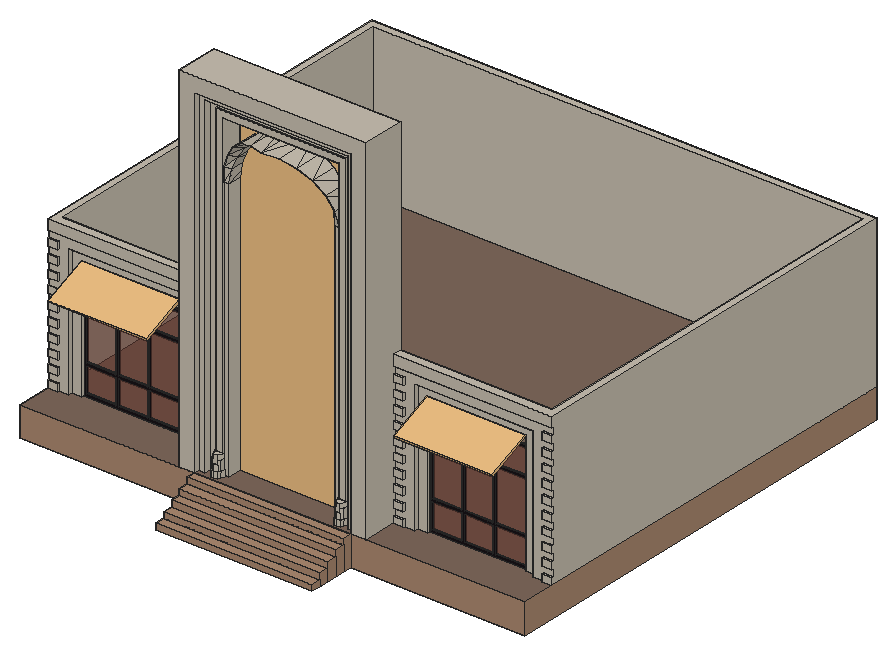
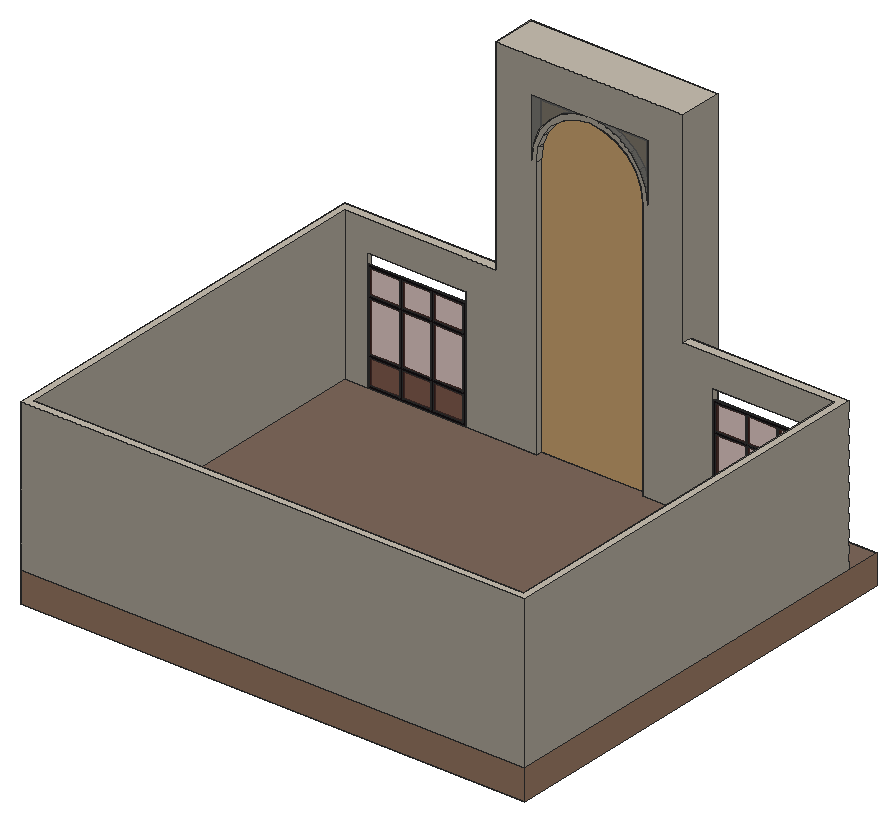
# SketchUp Ruby script. Lengths in inches.
U = 1.inch
M = Sketchup.active_model
def pt(a) = Geom::Point3d.new(a.map { |v| v * U })
def face(e, loops, mat)
  f = e.add_face(loops[0].map { |a| pt(a) })
  loops[1..].each { |l| e.add_face(l.map { |a| pt(a) }).erase! }
  f.material = f.back_material = mat if mat
  f
end
# faces: each face lists its corners as indices into pts; further lists are holes
def faces(e, pts, list, mat = nil) = list.each { |f| face(e, (f[0].is_a?(Array) ? f : [f]).map { |l| l.map { |i| pts[i] } }, mat) }
# xy, xz, yz: faces in a plane at the given z, y or x. An outline is a flat list of corners, or four numbers for a rectangle; further outlines are holes
def ring(l) = l.size == 4 ? [[l[0], l[1]], [l[2], l[1]], [l[2], l[3]], [l[0], l[3]]] : l.each_slice(2).to_a
def flat(e, list, mat, &to3) = list.each { |f| face(e, (f[0].is_a?(Array) ? f : [f]).map { |l| ring(l).map { |u, v| to3.(u, v) } }, mat) }
def xy(e, z, list, mat = nil) = flat(e, list, mat) { |x, y| [x, y, z] }
def xz(e, y, list, mat = nil) = flat(e, list, mat) { |x, z| [x, y, z] }
def yz(e, x, list, mat = nil) = flat(e, list, mat) { |y, z| [x, y, z] }
def lines(e, pts, list) = list.each { |a, b| e.add_line(pt(pts[a]), pt(pts[b])) }
# prism: a flat outline (further loops are holes) pulled along v
def prism(e, loops, v, mat = nil)
  f = face(e, loops, mat); d = Geom::Vector3d.new(v.map { |x| x * U })
  f.pushpull(f.normal.samedirection?(d) ? d.length : -d.length)
end
def box(e, o, s, mat = nil) = prism(e, [[o, [o[0] + s[0], o[1], o[2]], [o[0] + s[0], o[1] + s[1], o[2]], [o[0], o[1] + s[1], o[2]]]], [0, 0, s[2]], mat)
def at(x, y, z, deg = 0) = Geom::Transformation.translation(pt([x, y, z])) * Geom::Transformation.rotation(ORIGIN, Z_AXIS, deg.degrees)
def axes(o, x, y, z) = Geom::Transformation.new([*x, 0, *y, 0, *z, 0, *pt(o).to_a, 1])
def part(name) = M.definitions.add(name)
# library, detail: a bought-in or finely detailed component or shape, given as its bounding box
def library(name, o, s) = part(name).tap { |d| box(d.entities, o, s) }
def detail(e, o, s) = box(e.add_group.entities, o, s)
def put(e, d, t, mat = nil) = e.add_instance(d, t).tap { |i| i.material = mat if mat }
def group(e, t, mat = nil) = e.add_group.tap { |g| g.transformation = t; g.material = mat if mat }.entities
root = M.entities
M.materials.add("[0034_Wheat]").color = [198, 190, 175]
M.materials.add("[Color M06]").color = [86, 86, 86]
M.materials.add("[Color M07]").color = [25, 20, 24]
M.materials.add("[Granite Brown]").color = [126, 104, 91]
M.materials.add("[Tile Veriegated Stone]").color = [171, 137, 112]
M.materials.add("[Translucent Glass Block Dark]").color = [124, 124, 121]
M.materials["[Translucent Glass Block Dark]"].alpha = 0.8
M.materials.add("[Translucent Glass Dark Green]").color = [114, 59, 48]
M.materials["[Translucent Glass Dark Green]"].alpha = 0.5
c1 = part("Generic Models 17 - Generic Models 17-285328-_3D_")
xy(c1.entities,-17.72,[[-29.13,-33.15,-28.73,33.15,-16.92,33.15,-17.32,-33.15],[-17.32,-33.15,-16.92,33.15,-5.11,33.15,-5.51,-33.15],[-5.51,-33.15,-5.11,33.15,6.7,33.15,6.3,-33.15],[6.3,-33.15,6.7,33.15,18.51,33.15,18.12,-33.15],[18.12,-33.15,18.51,33.15,29.13,33.15,28.73,-33.15]],"[Tile Veriegated Stone]")
xy(c1.entities,-10.63,[[-29.13,-33.15,-17.32,-33.15,-16.92,33.15,-28.73,33.15]],"[Tile Veriegated Stone]")
xy(c1.entities,-3.54,[[-17.32,-33.15,-5.51,-33.15,-5.11,33.15,-16.92,33.15]],"[Tile Veriegated Stone]")
xy(c1.entities,3.54,[[-5.51,-33.15,6.3,-33.15,6.7,33.15,-5.11,33.15]],"[Tile Veriegated Stone]")
xy(c1.entities,10.63,[[6.3,-33.15,18.12,-33.15,18.51,33.15,6.7,33.15]],"[Tile Veriegated Stone]")
xy(c1.entities,17.72,[[18.12,-33.15,28.73,-33.15,29.13,33.15,18.51,33.15]],"[Tile Veriegated Stone]")
xz(c1.entities,-33.15,[[-29.13,-17.72,-17.32,-10.63],[-17.32,-17.72,-5.51,-3.54],[-5.51,-17.72,6.3,3.54],[6.3,-17.72,18.12,10.63],[18.12,-17.72,28.73,17.72]],"[Tile Veriegated Stone]")
xz(c1.entities,33.15,[[-28.73,-17.72,-16.92,-10.63],[-16.92,-17.72,-5.11,-3.54],[-5.11,-17.72,6.7,3.54],[6.7,-17.72,18.51,10.63],[18.51,-17.72,29.13,17.72]],"[Tile Veriegated Stone]")
p = [[-28.73,33.15,-10.63],[-28.73,33.15,-17.72],[-29.13,-33.15,-17.72],[-29.13,-33.15,-10.63],[-16.92,33.15,-3.54],[-16.92,33.15,-17.72],
  [-17.32,-33.15,-17.72],[-17.32,-33.15,-3.54],[-17.32,-33.15,-10.63],[-16.92,33.15,-10.63],[-5.11,33.15,3.54],[-5.11,33.15,-17.72],
  [-5.51,-33.15,-17.72],[-5.51,-33.15,3.54],[-5.51,-33.15,-3.54],[-5.11,33.15,-3.54],[6.7,33.15,10.63],[6.7,33.15,-17.72],
  [6.3,-33.15,-17.72],[6.3,-33.15,10.63],[6.3,-33.15,3.54],[6.7,33.15,3.54],[18.51,33.15,17.72],[18.51,33.15,-17.72],
  [18.12,-33.15,-17.72],[18.12,-33.15,17.72],[18.12,-33.15,10.63],[18.51,33.15,10.63],[28.73,-33.15,17.72],[28.73,-33.15,-17.72],
  [29.13,33.15,-17.72],[29.13,33.15,17.72]]
faces(c1.entities,p,[[0,1,2,3],[4,5,6,7],[8,6,5,9],[10,11,12,13],[14,12,11,15],[16,17,18,19],[20,18,17,21],[22,23,24,25],
  [26,24,23,27],[28,29,30,31]],"[Tile Veriegated Stone]")
c2 = part("Component\#1")
xy(c2.entities,0,[[3.83,0.21,5.3,1.0625,6.77,1.91,6.77,3.61,7.43,3.61,6.77,1.91,6.25,0.58]])
xy(c2.entities,7.0625,[[2.42,0,3.83,0.21,2.36,1.0625,0.89,1.91],[3.83,0.21,6.25,0.58,6.77,1.91,7.43,3.61,6.77,3.61,6.77,1.91,5.3,1.0625]])
xy(c2.entities,11.3125,[[0.89,1.91,0.89,3.61,0.23,3.61,0,3.03]])
xy(c2.entities,13.625,[[3.83,0.21,5.3,1.0625,2.36,1.0625]])
xy(c2.entities,18,[[2.36,1.0625,0.89,3.61,0.89,1.91],[5.3,1.0625,6.77,1.91,6.77,3.61]])
xy(c2.entities,24,[[2.36,1.0625,5.3,1.0625,6.77,3.61,0.89,3.61]])
xz(c2.entities,1.0625,[[2.36,13.625,5.3,24]])
xz(c2.entities,3.61,[[0.23,0,0.89,11.3125],[0.89,0,6.77,24],[6.77,0,7.43,7.0625]])
yz(c2.entities,0.89,[[1.91,11.3125,3.61,18]])
yz(c2.entities,6.77,[[1.91,7.0625,3.61,18]])
p = [[0.89,1.91,0],[2.42,0,0],[2.42,0,7.0625],[0.89,1.91,7.0625],[3.83,0.21,0],[3.83,0.21,7.0625],
  [6.25,0.58,0],[6.25,0.58,7.0625],[6.77,1.91,0],[6.77,1.91,7.0625],[0,3.03,0],[0.89,1.91,11.3125],
  [0,3.03,11.3125],[7.43,3.61,0],[7.43,3.61,7.0625],[0.23,3.61,0],[0.23,3.61,11.3125],[2.36,1.0625,13.625],
  [2.36,1.0625,7.0625],[3.83,0.21,13.625],[5.3,1.0625,7.0625],[5.3,1.0625,13.625],[2.36,1.0625,18],[0.89,1.91,18],
  [6.77,1.91,18],[5.3,1.0625,18],[0.89,3.61,24],[0.89,3.61,18],[2.36,1.0625,24],[5.3,1.0625,24],
  [6.77,3.61,18],[6.77,3.61,24],[5.3,1.0625,0]]
faces(c2.entities,p,[[0,1,2,3],[1,4,5,2],[4,6,7,5],[6,8,9,7],[10,0,3,11,12],[8,13,14,9],[15,10,12,16],[17,18,5,19],
  [19,5,20,21],[11,3,18,17,22,23],[21,20,9,24,25],[26,27,22,28],[29,25,30,31]])
lines(c2.entities,p,[[32,20]])
c3 = part("window")
xy(c3.entities,0,[[0,0,117,2]])
xy(c3.entities,3,[[3,0,38.5,2],[38.5,0,41.5,2],[41.5,0,75.5,2],[75.5,0,78.5,2],[78.5,0,114,2]])
xy(c3.entities,33,[[3,0,38.5,2],[41.5,0,75.5,2],[78.5,0,114,2]])
xy(c3.entities,36,[[3,0,38.5,2],[41.5,0,75.5,2],[78.5,0,114,2]])
xy(c3.entities,96,[[3,0,38.5,2],[41.5,0,75.5,2],[78.5,0,114,2]])
xy(c3.entities,99,[[3,0,38.5,2],[41.5,0,75.5,2],[78.5,0,114,2]])
xy(c3.entities,129,[[3,0,38.5,2],[41.5,0,75.5,2],[78.5,0,114,2]])
xy(c3.entities,132,[[0,0,117,2]])
xz(c3.entities,0,[[[0,0,117,132],[3,3,3,33,38.5,33,38.5,3,41.5,3,41.5,33,75.5,33,75.5,3,78.5,3,78.5,33,114,33,114,3],[3,36,38.5,96],[78.5,36,114,96],[41.5,36,75.5,96],[78.5,99,114,129],[3,99,38.5,129],[41.5,99,75.5,129]]])
xz(c3.entities,2,[[[0,0,117,132],[3,3,114,3,114,33,78.5,33,78.5,3,75.5,3,75.5,33,41.5,33,41.5,3,38.5,3,38.5,33,3,33],[3,36,38.5,96],[78.5,36,114,96],[41.5,36,75.5,96],[78.5,99,114,129],[3,99,38.5,129],[41.5,99,75.5,129]]])
xz(c3.entities,2,[[3,3,38.5,33],[41.5,3,75.5,33],[78.5,3,114,33],[3,36,38.5,96],[41.5,36,75.5,96],
  [78.5,36,114,96],[3,99,38.5,129],[41.5,99,75.5,129],[78.5,99,114,129]],"[Translucent Glass Dark Green]")
yz(c3.entities,0,[[0,0,2,132]])
yz(c3.entities,3,[[0,3,2,33],[0,36,2,96],[0,99,2,129]])
yz(c3.entities,38.5,[[0,3,2,33],[0,36,2,96],[0,99,2,129]])
yz(c3.entities,41.5,[[0,3,2,33],[0,36,2,96],[0,99,2,129]])
yz(c3.entities,75.5,[[0,3,2,33],[0,36,2,96],[0,99,2,129]])
yz(c3.entities,78.5,[[0,3,2,33],[0,36,2,96],[0,99,2,129]])
yz(c3.entities,114,[[0,3,2,33],[0,36,2,96],[0,99,2,129]])
yz(c3.entities,117,[[0,0,2,132]])
c4 = library("Group\#4",[8,99.8125,8],[126,14,375])
c5 = library("Group\#57",[0,-0.05,0],[53.97,2.25,80.01])
put(root,c1,axes([348,29.87,6.28],[0,1,0],[-2.8057,0,0],[0,0,1]),"[Tile Veriegated Stone]")
g1 = group(root,at(48,-18.57,0),"[Tile Veriegated Stone]")
xy(g1,-11.43,[[0,77.5625,600,600]])
xy(g1,24,[[0,77.5625,600,600]],"[Granite Brown]")
xz(g1,77.5625,[[0,-11.43,600,24]])
xz(g1,600,[[0,-11.43,600,24]])
yz(g1,0,[[77.5625,-11.43,600,24]])
yz(g1,600,[[77.5625,-11.43,600,24]])
g2 = group(root,at(48,101.43,24),"[0034_Wheat]")
xy(g2,0,[[189,-42.4375,189,-2,177,-2,177,0,165,0,165,4,153,4,153,9,237,9,237,-29,231,-29,231,-30,223,-30,223,-29,215,-29,215,-36.1875,207,-36.1875,207,-42.4375],[393,-42.4375,393,-36.1875,385,-36.1875,385,-29,377,-29,377,-30,369,-30,369,-29,363,-29,363,9,447,9,447,4,435,4,435,0,423,0,423,-2,411,-2,411,-42.4375],[0,-2,0,480,600,480,600,-2,588,-2,588,0,576,0,576,4,564,4,564,9,591,9,591,471,9,471,9,9,36,9,36,4,24,4,24,0,12,0,12,-2]])
xy(g2,8.4,[[0,-2,12,0],[177,-2,189,0],[411,-2,423,0],[588,-2,600,0]])
xy(g2,16.8,[[0,-2,12,0],[177,-2,189,0],[411,-2,423,0],[588,-2,600,0]])
xy(g2,25.2,[[0,-2,12,0],[177,-2,189,0],[411,-2,423,0],[588,-2,600,0]])
xy(g2,33.6,[[0,-2,12,0],[177,-2,189,0],[411,-2,423,0],[588,-2,600,0]])
xy(g2,42,[[0,-2,12,0],[177,-2,189,0],[411,-2,423,0],[588,-2,600,0]])
xy(g2,50.4,[[0,-2,12,0],[177,-2,189,0],[411,-2,423,0],[588,-2,600,0]])
xy(g2,58.8,[[0,-2,12,0],[177,-2,189,0],[411,-2,423,0],[588,-2,600,0]])
xy(g2,67.2,[[0,-2,12,0],[177,-2,189,0],[411,-2,423,0],[588,-2,600,0]])
xy(g2,75.6,[[0,-2,12,0],[177,-2,189,0],[411,-2,423,0],[588,-2,600,0]])
xy(g2,84,[[0,-2,12,0],[177,-2,189,0],[411,-2,423,0],[588,-2,600,0]])
xy(g2,92.4,[[0,-2,12,0],[177,-2,189,0],[411,-2,423,0],[588,-2,600,0]])
xy(g2,100.8,[[0,-2,12,0],[177,-2,189,0],[411,-2,423,0],[588,-2,600,0]])
xy(g2,109.2,[[0,-2,12,0],[177,-2,189,0],[411,-2,423,0],[588,-2,600,0]])
xy(g2,117.6,[[0,-2,12,0],[177,-2,189,0],[411,-2,423,0],[588,-2,600,0]])
xy(g2,126,[[0,-2,12,0],[177,-2,189,0],[411,-2,423,0],[588,-2,600,0]])
xy(g2,134.4,[[0,-2,12,0],[177,-2,189,0],[411,-2,423,0],[588,-2,600,0]])
xy(g2,142.8,[[0,-2,12,0],[177,-2,189,0],[411,-2,423,0],[588,-2,600,0]])
xy(g2,144,[[36,4,153,9],[447,4,564,9]])
xy(g2,151.2,[[0,-2,12,0],[177,-2,189,0],[411,-2,423,0],[588,-2,600,0]])
xy(g2,156,[[24,0,165,4],[435,0,576,4]])
xy(g2,159.6,[[0,-2,12,0],[177,-2,189,0],[411,-2,423,0],[588,-2,600,0]])
xy(g2,168,[[0,-2,189,0],[411,-2,600,0]])
xy(g2,180,[[0,-2,189,-2,189,9,9,9,9,471,591,471,591,9,411,9,411,-2,600,-2,600,480,0,480]])
xy(g2,381,[[231,-30,300,9],[300,-30,366.65,9],[366.65,-30,369,9]])
xy(g2,389,[[223,-30,377,-29]])
xy(g2,397,[[215,-36.1875,385,-29]])
xy(g2,405,[[207,-42.4375,393,-36.1875]])
xy(g2,423,[[189,-42.4375,411,9]])
xz(g2,-42.4375,[[189,0,207,0,207,405,393,405,393,0,411,0,411,423,189,423]])
xz(g2,-36.1875,[[207,0,215,0,215,397,385,397,385,0,393,0,393,405,207,405]])
xz(g2,-30,[[223,0,231,0,231,381,369,381,369,0,377,0,377,389,223,389]])
xz(g2,-29,[[215,0,223,0,223,389,377,389,377,0,385,0,385,397,215,397],[231,0,237,312],[363,0,369,312]])
xz(g2,-2,[[0,0,12,8.4],[177,0,189,8.4],[411,0,423,8.4],[588,0,600,8.4],[0,16.8,12,25.2],
  [177,16.8,189,25.2],[411,16.8,423,25.2],[588,16.8,600,25.2],[0,33.6,12,42],[177,33.6,189,42],
  [411,33.6,423,42],[588,33.6,600,42],[0,50.4,12,58.8],[177,50.4,189,58.8],[411,50.4,423,58.8],
  [588,50.4,600,58.8],[0,67.2,12,75.6],[177,67.2,189,75.6],[411,67.2,423,75.6],[588,67.2,600,75.6],
  [0,84,12,92.4],[177,84,189,92.4],[411,84,423,92.4],[588,84,600,92.4],[0,100.8,12,109.2],
  [177,100.8,189,109.2],[411,100.8,423,109.2],[588,100.8,600,109.2],[0,117.6,12,126],[177,117.6,189,126],
  [411,117.6,423,126],[588,117.6,600,126],[0,134.4,12,142.8],[177,134.4,189,142.8],[411,134.4,423,142.8],
  [588,134.4,600,142.8],[0,151.2,12,159.6],[177,151.2,189,159.6],[411,151.2,423,159.6],[588,151.2,600,159.6],
  [0,168,189,180],[411,168,600,180]])
xz(g2,0,[[12,0,24,0,24,156,165,156,165,0,177,0,177,8.4,189,8.4,189,16.8,177,16.8,177,25.2,189,25.2,189,33.6,177,33.6,177,42,189,42,189,50.4,177,50.4,177,58.8,189,58.8,189,67.2,177,67.2,177,75.6,189,75.6,189,84,177,84,177,92.4,189,92.4,189,100.8,177,100.8,177,109.2,189,109.2,189,117.6,177,117.6,177,126,189,126,189,134.4,177,134.4,177,142.8,189,142.8,189,151.2,177,151.2,177,159.6,189,159.6,189,168,0,168,0,159.6,12,159.6,12,151.2,0,151.2,0,142.8,12,142.8,12,134.4,0,134.4,0,126,12,126,12,117.6,0,117.6,0,109.2,12,109.2,12,100.8,0,100.8,0,92.4,12,92.4,12,84,0,84,0,75.6,12,75.6,12,67.2,0,67.2,0,58.8,12,58.8,12,50.4,0,50.4,0,42,12,42,12,33.6,0,33.6,0,25.2,12,25.2,12,16.8,0,16.8,0,8.4,12,8.4],[423,0,435,0,435,156,576,156,576,0,588,0,588,8.4,600,8.4,600,16.8,588,16.8,588,25.2,600,25.2,600,33.6,588,33.6,588,42,600,42,600,50.4,588,50.4,588,58.8,600,58.8,600,67.2,588,67.2,588,75.6,600,75.6,600,84,588,84,588,92.4,600,92.4,600,100.8,588,100.8,588,109.2,600,109.2,600,117.6,588,117.6,588,126,600,126,600,134.4,588,134.4,588,142.8,600,142.8,600,151.2,588,151.2,588,159.6,600,159.6,600,168,411,168,411,159.6,423,159.6,423,151.2,411,151.2,411,142.8,423,142.8,423,134.4,411,134.4,411,126,423,126,423,117.6,411,117.6,411,109.2,423,109.2,423,100.8,411,100.8,411,92.4,423,92.4,423,84,411,84,411,75.6,423,75.6,423,67.2,411,67.2,411,58.8,423,58.8,423,50.4,411,50.4,411,42,423,42,423,33.6,411,33.6,411,25.2,423,25.2,423,16.8,411,16.8,411,8.4,423,8.4]])
xz(g2,4,[[24,0,36,0,36,144,153,144,153,0,165,0,165,156,24,156],[435,0,447,0,447,144,564,144,564,0,576,0,576,156,435,156]])
xz(g2,9,[[[9,0,9,180,189,180,189,423,411,423,411,180,591,180,591,0,564,0,564,144,447,144,447,0,363,0,363,312,360.85,328.31,354.56,343.5,344.55,356.55,331.5,366.56,316.31,372.85,300,375,283.69,372.85,268.5,366.56,255.45,356.55,245.44,343.5,239.15,328.31,237,312,237,0,153,0,153,144,36,144,36,0],[369,312,369,381,300,381,317.86,378.65,334.5,371.76,348.79,360.79,359.76,346.5,366.65,329.86],[231,312,233.35,329.86,240.24,346.5,251.21,360.79,265.5,371.76,282.14,378.65,300,381,231,381]]])
xz(g2,471,[[9,0,591,180]])
xz(g2,480,[[0,0,600,180]])
yz(g2,0,[[-2,0,-2,8.4,0,8.4,0,16.8,-2,16.8,-2,25.2,0,25.2,0,33.6,-2,33.6,-2,42,0,42,0,50.4,-2,50.4,-2,58.8,0,58.8,0,67.2,-2,67.2,-2,75.6,0,75.6,0,84,-2,84,-2,92.4,0,92.4,0,100.8,-2,100.8,-2,109.2,0,109.2,0,117.6,-2,117.6,-2,126,0,126,0,134.4,-2,134.4,-2,142.8,0,142.8,0,151.2,-2,151.2,-2,159.6,0,159.6,0,168,-2,168,-2,180,480,180,480,0]])
yz(g2,9,[[9,0,471,180]])
yz(g2,12,[[-2,0,0,8.4],[-2,16.8,0,25.2],[-2,33.6,0,42],[-2,50.4,0,58.8],[-2,67.2,0,75.6],
  [-2,84,0,92.4],[-2,100.8,0,109.2],[-2,117.6,0,126],[-2,134.4,0,142.8],[-2,151.2,0,159.6]])
yz(g2,24,[[0,0,4,156]])
yz(g2,36,[[4,0,9,144]])
yz(g2,153,[[4,0,9,144]])
yz(g2,165,[[0,0,4,156]])
yz(g2,177,[[-2,0,0,8.4],[-2,16.8,0,25.2],[-2,33.6,0,42],[-2,50.4,0,58.8],[-2,67.2,0,75.6],
  [-2,84,0,92.4],[-2,100.8,0,109.2],[-2,117.6,0,126],[-2,134.4,0,142.8],[-2,151.2,0,159.6]])
yz(g2,189,[[-42.4375,0,-42.4375,423,9,423,9,180,-2,180,-2,168,0,168,0,159.6,-2,159.6,-2,151.2,0,151.2,0,142.8,-2,142.8,-2,134.4,0,134.4,0,126,-2,126,-2,117.6,0,117.6,0,109.2,-2,109.2,-2,100.8,0,100.8,0,92.4,-2,92.4,-2,84,0,84,0,75.6,-2,75.6,-2,67.2,0,67.2,0,58.8,-2,58.8,-2,50.4,0,50.4,0,42,-2,42,-2,33.6,0,33.6,0,25.2,-2,25.2,-2,16.8,0,16.8,0,8.4,-2,8.4,-2,0]])
yz(g2,207,[[-42.4375,0,-36.1875,405]])
yz(g2,215,[[-36.1875,0,-29,397]])
yz(g2,223,[[-30,0,-29,389]])
yz(g2,231,[[-30,0,-29,0,-29,312,9,312,9,381,-30,381]])
yz(g2,237,[[-29,0,9,312]])
yz(g2,363,[[-29,0,9,312]])
yz(g2,369,[[-30,0,-29,312],[-30,312,9,381]])
yz(g2,377,[[-30,0,-29,389]])
yz(g2,385,[[-36.1875,0,-29,397]])
yz(g2,393,[[-42.4375,0,-36.1875,405]])
yz(g2,411,[[-42.4375,0,-2,0,-2,8.4,0,8.4,0,16.8,-2,16.8,-2,25.2,0,25.2,0,33.6,-2,33.6,-2,42,0,42,0,50.4,-2,50.4,-2,58.8,0,58.8,0,67.2,-2,67.2,-2,75.6,0,75.6,0,84,-2,84,-2,92.4,0,92.4,0,100.8,-2,100.8,-2,109.2,0,109.2,0,117.6,-2,117.6,-2,126,0,126,0,134.4,-2,134.4,-2,142.8,0,142.8,0,151.2,-2,151.2,-2,159.6,0,159.6,0,168,-2,168,-2,180,9,180,9,423,-42.4375,423]])
yz(g2,423,[[-2,0,0,8.4],[-2,16.8,0,25.2],[-2,33.6,0,42],[-2,50.4,0,58.8],[-2,67.2,0,75.6],
  [-2,84,0,92.4],[-2,100.8,0,109.2],[-2,117.6,0,126],[-2,134.4,0,142.8],[-2,151.2,0,159.6]])
yz(g2,435,[[0,0,4,156]])
yz(g2,447,[[4,0,9,144]])
yz(g2,564,[[4,0,9,144]])
yz(g2,576,[[0,0,4,156]])
yz(g2,588,[[-2,0,0,8.4],[-2,16.8,0,25.2],[-2,33.6,0,42],[-2,50.4,0,58.8],[-2,67.2,0,75.6],
  [-2,84,0,92.4],[-2,100.8,0,109.2],[-2,117.6,0,126],[-2,134.4,0,142.8],[-2,151.2,0,159.6]])
yz(g2,591,[[9,0,471,180]])
yz(g2,600,[[-2,0,480,0,480,180,-2,180,-2,168,0,168,0,159.6,-2,159.6,-2,151.2,0,151.2,0,142.8,-2,142.8,-2,134.4,0,134.4,0,126,-2,126,-2,117.6,0,117.6,0,109.2,-2,109.2,-2,100.8,0,100.8,0,92.4,-2,92.4,-2,84,0,84,0,75.6,-2,75.6,-2,67.2,0,67.2,0,58.8,-2,58.8,-2,50.4,0,50.4,0,42,-2,42,-2,33.6,0,33.6,0,25.2,-2,25.2,-2,16.8,0,16.8,0,8.4,-2,8.4]])
p = [[360.85,-27.55,328.24],[363,-29,312],[367.02,-33.48,330.23],[369,-29,312],[366.65,0,329.86],[233.59,-31.4,330.54],
  [233.35,2,329.86],[231,-29,312],[239.15,-27.55,328.24],[237,-29,312],[231,2,312],[239.15,9,328.31],
  [237,9,312],[360.85,9,328.31],[363,9,312],[369,0,312],[369,9,312],[366.65,9,329.86],
  [233.35,9,329.86],[231,9,312],[354.56,-26.2,343.375],[245.44,-26.2,343.375],[354.56,9,343.5],[245.44,9,343.5],
  [359.76,0,346.5],[360.36,-38.6875,347.1],[240.24,2,346.5],[359.76,9,346.5],[240.24,9,346.5],[240.625,-35.3125,347.61],
  [344.55,-25.04,356.37],[255.45,-25.04,356.37],[344.55,9,356.55],[255.45,9,356.55],[348.79,0,360.79],[349.47,-44.28,361.47],
  [251.21,2,360.79],[348.79,9,360.79],[251.21,9,360.79],[251.64,-40.46,362.05],[331.5,-24.16,366.34],[268.5,-24.16,366.34],
  [268.5,9,366.56],[331.5,9,366.56],[265.88,-46.5,372.87],[265.5,2,371.76],[334.5,0,371.76],[334.5,9,371.76],
  [265.5,9,371.76],[335.1,-49.875,372.36],[316.31,-23.6,372.61],[283.69,-23.6,372.61],[283.69,9,372.85],[316.31,9,372.85],
  [282.375,-53.01,379.33],[282.14,2,378.65],[317.86,0,378.65],[317.86,9,378.65],[282.14,9,378.65],[318.23,-55.09,379.02],
  [300,-23.41,374.75],[300,9,375],[300,-59.5625,381],[300,-30,381],[300,0,381],[300,2,381],
  [300,9,381]]
faces(g2,p,[[0,1,2],[3,2,1],[4,2,3],[5,6,7],[5,7,8],[9,8,7],[7,6,10],[11,8,9],
  [12,11,9],[1,13,14],[0,13,1],[4,3,15],[4,15,16,17],[10,6,18,19],[20,0,2],[21,5,8],
  [8,11,21],[13,0,22],[20,22,0],[23,21,11],[24,25,4],[2,4,25],[6,5,26],[24,4,17,27],
  [6,26,28,18],[25,20,2],[29,26,5],[29,5,21],[30,20,25],[31,29,21],[21,23,31],[22,20,32],
  [30,32,20],[33,31,23],[34,35,24],[25,24,35],[26,29,36],[34,24,27,37],[26,36,38,28],[35,30,25],
  [39,36,29],[39,29,31],[40,30,35],[41,39,31],[33,42,31],[41,31,42],[30,40,32],[43,32,40],
  [39,44,36],[45,36,44],[34,46,35],[46,34,37,47],[36,45,48,38],[49,40,35],[49,35,46],[44,39,41],
  [50,40,49],[51,44,41],[42,52,41],[51,41,52],[40,50,43],[53,43,50],[44,54,45],[55,45,54],
  [46,56,49],[56,46,47,57],[45,55,58,48],[59,50,49],[59,49,56],[60,50,59],[54,44,51],[60,54,51],
  [52,61,51],[60,51,61],[50,60,53],[61,53,60],[54,60,59],[54,62,55],[62,63,64,65,55],[59,56,62],
  [63,62,56,64],[64,56,57,66,65],[55,65,66,58],[62,54,59]])
put(g2,c2,axes([219.76,-39.33,0],[1.8908,0,0],[0,2.584,0],[0,0,1]))
put(g2,c2,axes([365.76,-39.33,0],[1.8908,0,0],[0,2.584,0],[0,0,1]))
g3 = group(g2,at(231,9,312),"[Translucent Glass Block Dark]")
xz(g3,0,[[0,0,0,69,69,69,51.14,66.65,34.5,59.76,20.21,48.79,9.24,34.5,2.35,17.86],[138,0,135.65,17.86,128.76,34.5,117.79,48.79,103.5,59.76,86.86,66.65,69,69,138,69]])
put(root,c3,at(84,108.43,24),"[Color M07]")
put(root,c3,at(495,108.43,24),"[Color M07]")
put(root,c4,at(277,-10.38,16),"[Color M07]")
put(root,c5,axes([201.01,55.12,148.76],[0,0.92239,0.38627],[-0.00389,0.38626,-0.92238],[-1.46245,-0.0022,0.00525]),"[Color M06]")
put(root,c5,axes([612.01,55.12,148.76],[0,0.92239,0.38627],[-0.00389,0.38626,-0.92238],[-1.46245,-0.0022,0.00525]),"[Color M06]")
